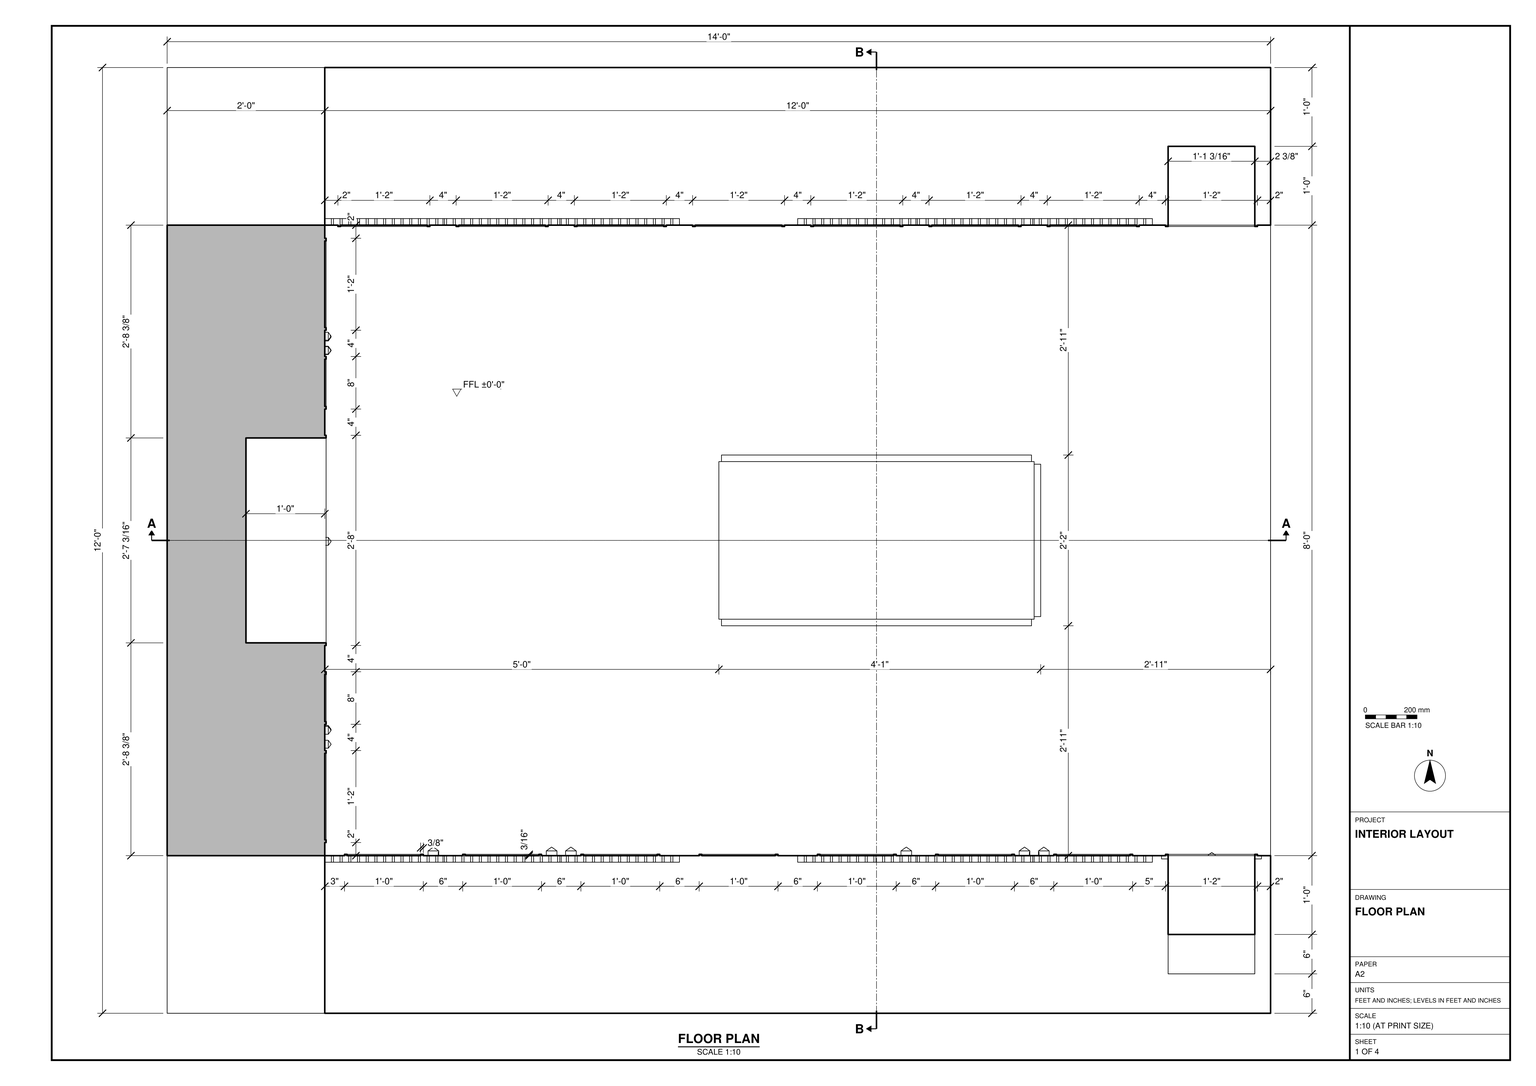
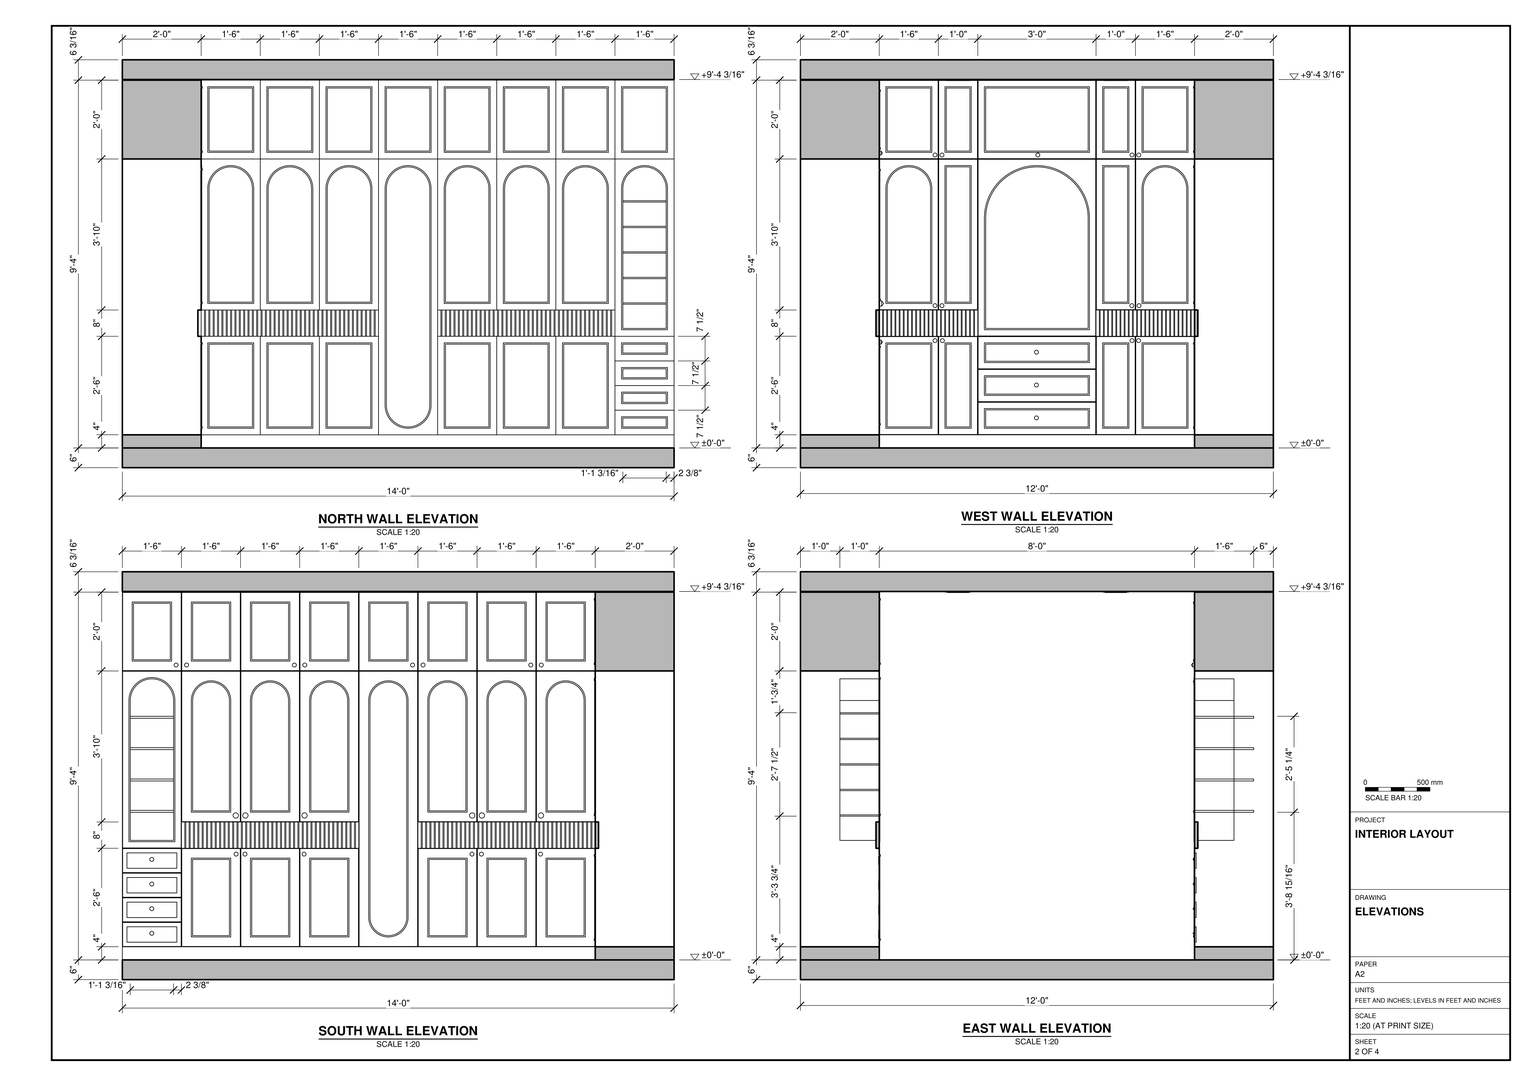
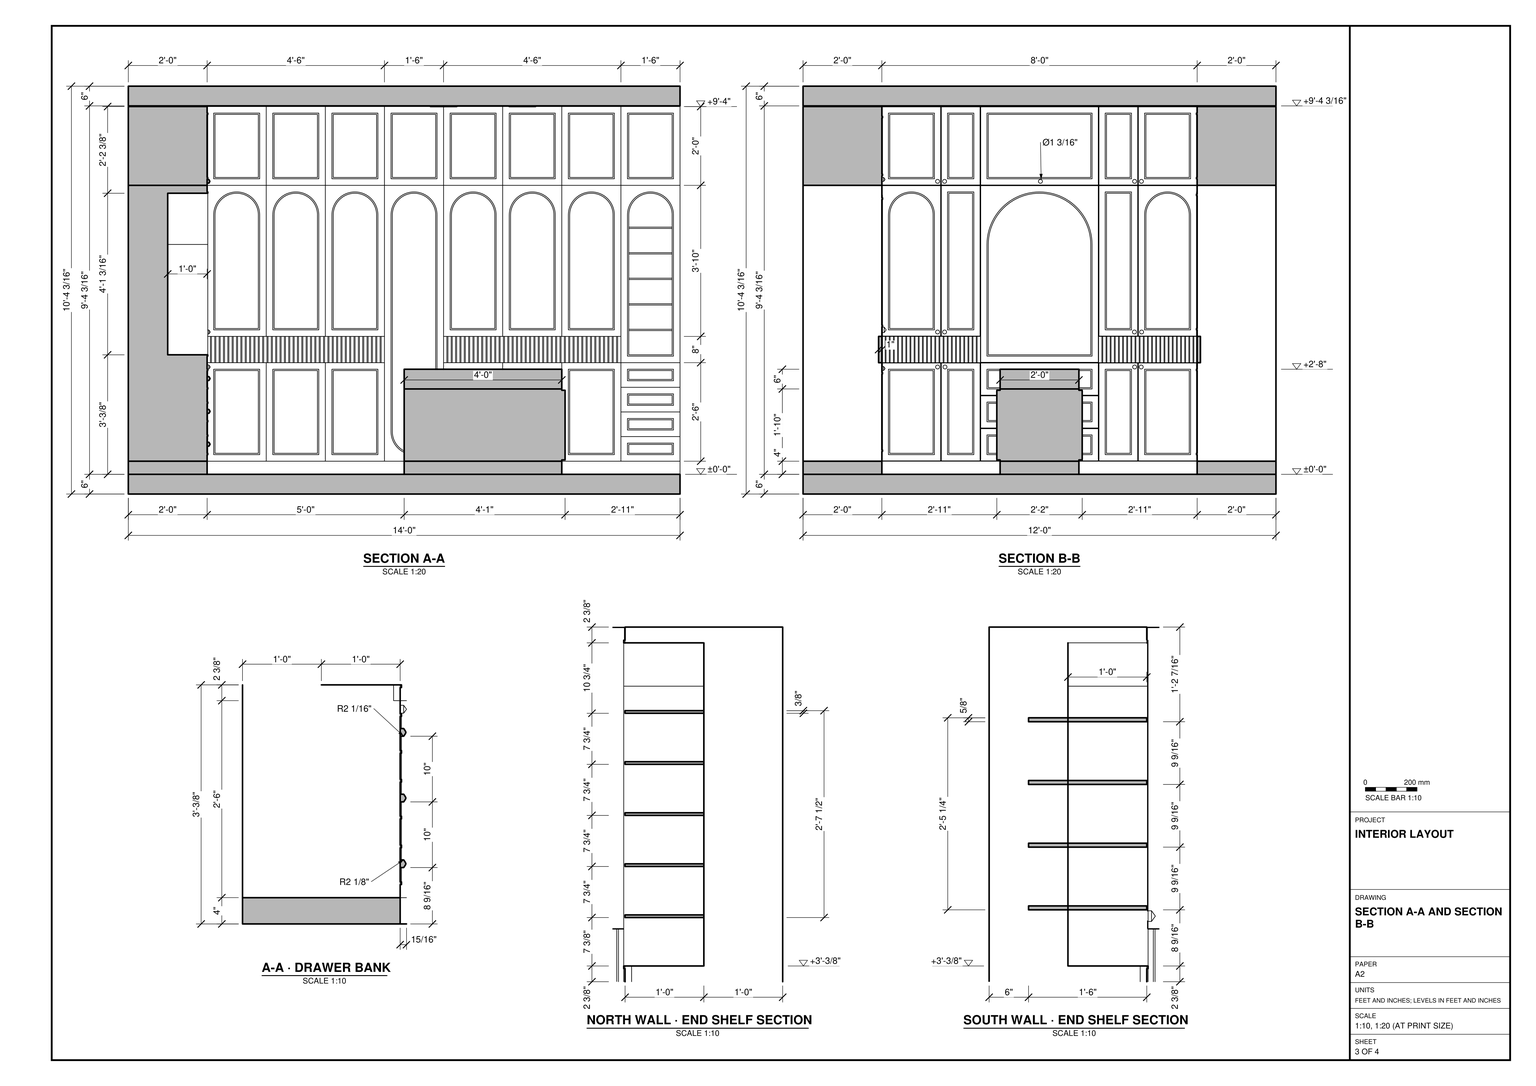
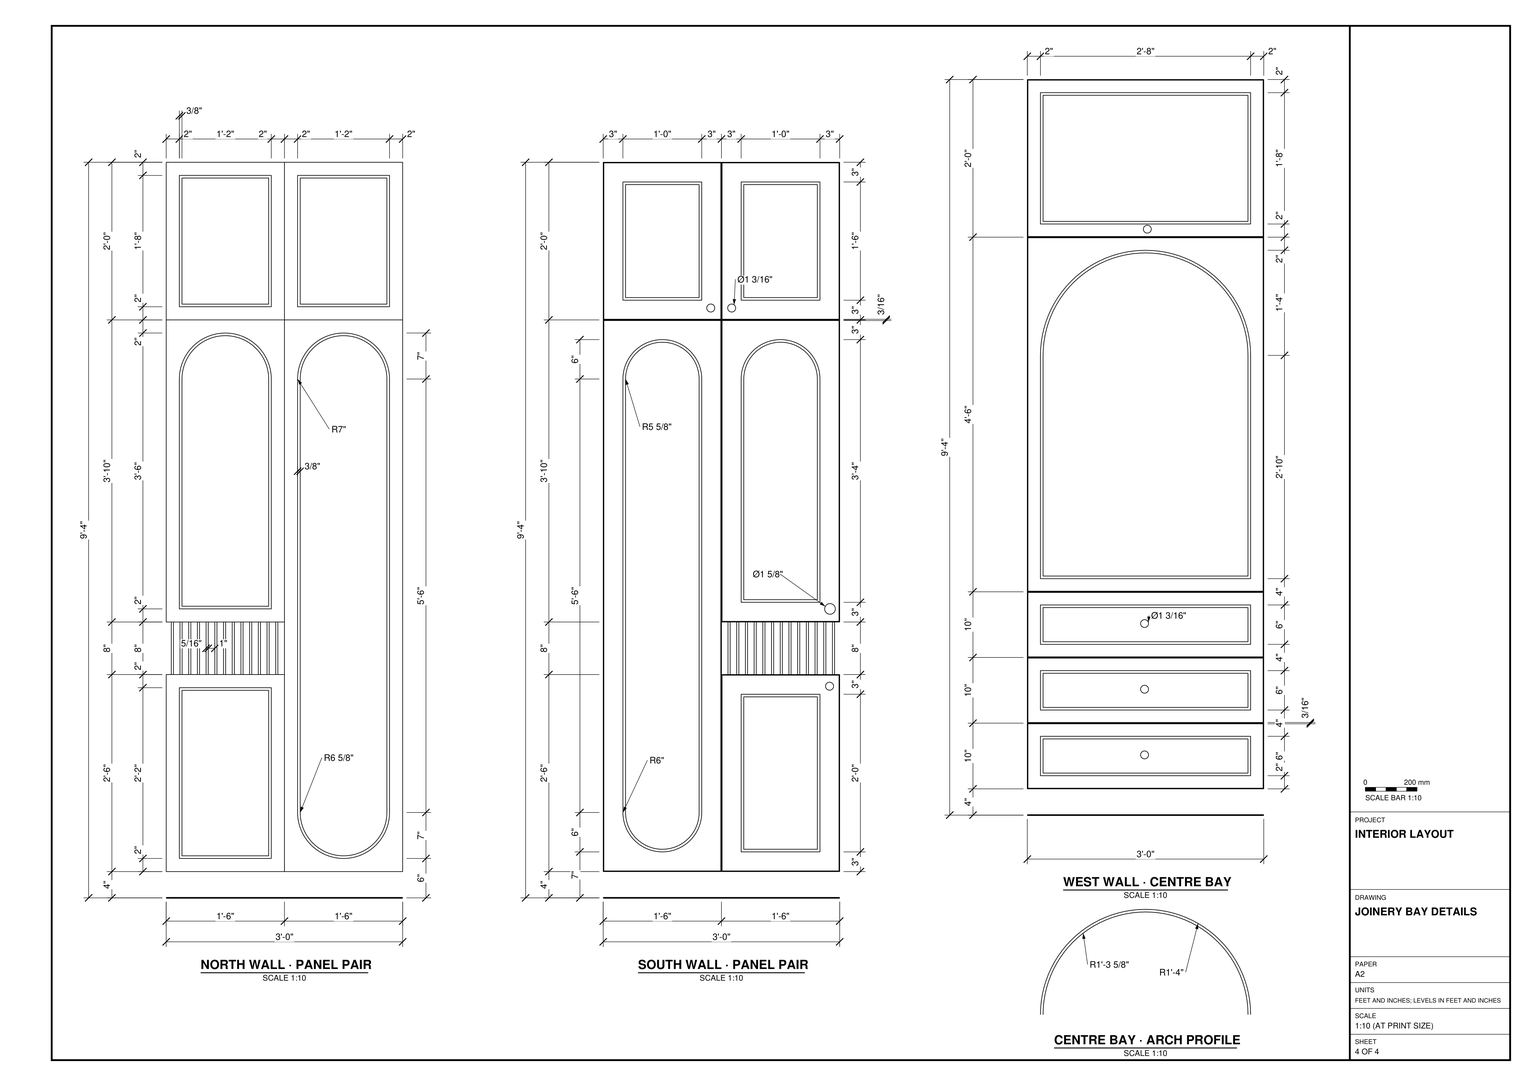
Build the dressing room in SketchUp from task_files/diagram_01.pdf. Work in feet and inches. The overall model is 14'-0" east to west, 12'-0" north to south and 10'-4 3/16" high. Use the single finished floor level of ±0'-0". Model the floor slab below that level and the ceiling slab above the cabinetry, following the thicknesses and edges in the sections.

Lay out the built-in storage along the north, south and west sides, leaving the east side clear between the ends of the long runs. On the north and south faces, align the upper cupboards, arched panels, ribbed bands and lower cupboards as shown in the elevations. Include the tall round-ended panel in each run and the shelved bay above a drawer stack at each east end. Follow the separate shelf sections rather than making the two end bays identical. On the west side, form the wider central arched recess over the drawer bank, with narrower cabinets to either side.

Model the freestanding island with its plinth, body and top. Use its overall footprint, rather than its plinth, to set the clearances shown in plan. Keep shell elements and individual furniture or joinery pieces in separate groups or components, and use components for repeated parts. Any decor or loose items shown may be suitable library components. Save one SketchUp model as output_files/walk_in_dressing_room_with_a_freestanding_island.skp.

# SketchUp Ruby script. Lengths in inches.
U = 1.inch
M = Sketchup.active_model
def pt(a) = Geom::Point3d.new(a.map { |v| v * U })
def face(e, loops, mat)
  f = e.add_face(loops[0].map { |a| pt(a) })
  loops[1..].each { |l| e.add_face(l.map { |a| pt(a) }).erase! }
  f.material = f.back_material = mat if mat
  f
end
# faces: each face lists its corners as indices into pts; further lists are holes
def faces(e, pts, list, mat = nil) = list.each { |f| face(e, (f[0].is_a?(Array) ? f : [f]).map { |l| l.map { |i| pts[i] } }, mat) }
# xy, xz, yz: faces in a plane at the given z, y or x. An outline is a flat list of corners, or four numbers for a rectangle; further outlines are holes
def ring(l) = l.size == 4 ? [[l[0], l[1]], [l[2], l[1]], [l[2], l[3]], [l[0], l[3]]] : l.each_slice(2).to_a
def flat(e, list, mat, &to3) = list.each { |f| face(e, (f[0].is_a?(Array) ? f : [f]).map { |l| ring(l).map { |u, v| to3.(u, v) } }, mat) }
def xy(e, z, list, mat = nil) = flat(e, list, mat) { |x, y| [x, y, z] }
def xz(e, y, list, mat = nil) = flat(e, list, mat) { |x, z| [x, y, z] }
def yz(e, x, list, mat = nil) = flat(e, list, mat) { |y, z| [x, y, z] }
def lines(e, pts, list) = list.each { |a, b| e.add_line(pt(pts[a]), pt(pts[b])) }
# prism: a flat outline (further loops are holes) pulled along v
def prism(e, loops, v, mat = nil)
  f = face(e, loops, mat); d = Geom::Vector3d.new(v.map { |x| x * U })
  f.pushpull(f.normal.samedirection?(d) ? d.length : -d.length)
end
def box(e, o, s, mat = nil) = prism(e, [[o, [o[0] + s[0], o[1], o[2]], [o[0] + s[0], o[1] + s[1], o[2]], [o[0], o[1] + s[1], o[2]]]], [0, 0, s[2]], mat)
def at(x, y, z, deg = 0) = Geom::Transformation.translation(pt([x, y, z])) * Geom::Transformation.rotation(ORIGIN, Z_AXIS, deg.degrees)
def axes(o, x, y, z) = Geom::Transformation.new([*x, 0, *y, 0, *z, 0, *pt(o).to_a, 1])
def part(name) = M.definitions.add(name)
# library, detail: a bought-in or finely detailed component or shape, given as its bounding box
def library(name, o, s) = part(name).tap { |d| box(d.entities, o, s) }
def detail(e, o, s) = box(e.add_group.entities, o, s)
def put(e, d, t, mat = nil) = e.add_instance(d, t).tap { |i| i.material = mat if mat }
def group(e, t, mat = nil) = e.add_group.tap { |g| g.transformation = t; g.material = mat if mat }.entities
root = M.entities
M.materials.add("[Translucent Glass Gray]1").color = [128, 128, 128]
M.materials.add("[Wood Veneer 01]").color = [104, 60, 32]
M.materials.add("download (3)").color = [228, 221, 207]
c1 = library("Group\#1",[0,0,0],[24.97,96,112])
c2 = part("Recessed ceiling light")
xy(c2.entities,0,[[4,0,2.96,0.14,2,0.54,1.17,1.17,0.54,2,0.14,2.96,0,4,0.14,5.04,0.54,6,1.17,6.83,2,7.46,2.96,7.86,4,8,5.04,7.86,6,7.46,6.83,6.83,7.46,6,7.86,5.04,8,4,7.86,2.96,7.46,2,6.83,1.17,6,0.54,5.04,0.14]])
xy(c2.entities,0.2,[[[4,0,5.04,0.14,6,0.54,6.83,1.17,7.46,2,7.86,2.96,8,4,7.86,5.04,7.46,6,6.83,6.83,6,7.46,5.04,7.86,4,8,2.96,7.86,2,7.46,1.17,6.83,0.54,6,0.14,5.04,0,4,0.14,2.96,0.54,2,1.17,1.17,2,0.54,2.96,0.14],[4,0.6,3.12,0.72,2.3,1.06,1.6,1.6,1.06,2.3,0.72,3.12,0.6,4,0.72,4.88,1.06,5.7,1.6,6.4,2.3,6.94,3.12,7.28,4,7.4,4.88,7.28,5.7,6.94,6.4,6.4,6.94,5.7,7.28,4.88,7.4,4,7.28,3.12,6.94,2.3,6.4,1.6,5.7,1.06,4.88,0.72]],[4,0.6,4.88,0.72,5.7,1.06,6.4,1.6,6.94,2.3,7.28,3.12,7.4,4,7.28,4.88,6.94,5.7,6.4,6.4,5.7,6.94,4.88,7.28,4,7.4,3.12,7.28,2.3,6.94,1.6,6.4,1.06,5.7,0.72,4.88,0.6,4,0.72,3.12,1.06,2.3,1.6,1.6,2.3,1.06,3.12,0.72]])
p = [[2.96,0.14,0],[4,0,0],[4,0,0.2],[2.96,0.14,0.2],[5.04,0.14,0],[5.04,0.14,0.2],
  [2,0.54,0],[2,0.54,0.2],[6,0.54,0],[6,0.54,0.2],[1.17,1.17,0],[1.17,1.17,0.2],
  [6.83,1.17,0],[6.83,1.17,0.2],[0.54,2,0],[0.54,2,0.2],[7.46,2,0],[7.46,2,0.2],
  [0.14,2.96,0],[0.14,2.96,0.2],[7.86,2.96,0],[7.86,2.96,0.2],[0,4,0],[0,4,0.2],
  [8,4,0],[8,4,0.2],[0.14,5.04,0],[0.14,5.04,0.2],[7.86,5.04,0],[7.86,5.04,0.2],
  [0.54,6,0],[0.54,6,0.2],[7.46,6,0],[7.46,6,0.2],[1.17,6.83,0],[1.17,6.83,0.2],
  [6.83,6.83,0],[6.83,6.83,0.2],[2,7.46,0],[2,7.46,0.2],[6,7.46,0],[6,7.46,0.2],
  [2.96,7.86,0],[2.96,7.86,0.2],[5.04,7.86,0],[5.04,7.86,0.2],[4,8,0],[4,8,0.2]]
faces(c2.entities,p,[[0,1,2,3],[1,4,5,2],[6,0,3,7],[4,8,9,5],[10,6,7,11],[8,12,13,9],[14,10,11,15],[12,16,17,13],
  [18,14,15,19],[16,20,21,17],[22,18,19,23],[20,24,25,21],[26,22,23,27],[24,28,29,25],[30,26,27,31],[28,32,33,29],
  [34,30,31,35],[32,36,37,33],[38,34,35,39],[36,40,41,37],[42,38,39,43],[40,44,45,41],[46,42,43,47],[44,46,47,45]])
c3 = part("Ceiling panel")
xy(c3.entities,0,[[0,0,0,144,168,144,168,120,24,120,24,24,168,24,168,0],[24,24,168,120]])
xy(c3.entities,6,[[0,0,168,144]])
xz(c3.entities,0,[[0,0,168,6]])
xz(c3.entities,144,[[0,0,168,6]])
yz(c3.entities,0,[[0,0,144,6]])
yz(c3.entities,168,[[0,0,144,6]])
c4 = library("Group\#18",[0,0,0],[144,24.2,112])
c5 = library("Group\#19",[0,0,0],[144,25.31,112])
put(root,c1,at(0,24,0))
g1 = group(root,at(84,60,0))
xy(g1,0,[[0,0,48,24]])
xy(g1,4,[[0,0,48,24]])
xy(g1,4.4,[[0.4,-1,47.6,0],[48,0.4,49,23.6],[0.4,24,47.6,25]],"[Wood Veneer 01]")
xy(g1,25.6,[[0.4,-1,47.6,0],[48,0.4,49,23.6],[0.4,24,47.6,25]],"[Wood Veneer 01]")
xy(g1,26,[[0,0,48,24]])
xy(g1,32,[[0,0,48,24]],"[Translucent Glass Gray]1")
xz(g1,-1,[[0.4,4.4,47.6,25.6]],"[Wood Veneer 01]")
xz(g1,0,[[0,26,48,32]],"[Translucent Glass Gray]1")
xz(g1,0,[[0,0,48,4],[[0,4,48,26],[0.4,4.4,47.6,25.6]]],"[Wood Veneer 01]")
xz(g1,0.4,[[48,4.4,49,25.6]],"[Wood Veneer 01]")
xz(g1,23.6,[[48,4.4,49,25.6]],"[Wood Veneer 01]")
xz(g1,24,[[0,26,48,32]],"[Translucent Glass Gray]1")
xz(g1,24,[[0,0,48,4],[[0,4,48,26],[0.4,4.4,47.6,25.6]]],"[Wood Veneer 01]")
xz(g1,25,[[0.4,4.4,47.6,25.6]],"[Wood Veneer 01]")
yz(g1,0,[[0,0,24,4],[0,4,24,26]])
yz(g1,0,[[0,26,24,32]],"[Translucent Glass Gray]1")
yz(g1,0.4,[[-1,4.4,0,25.6],[24,4.4,25,25.6]],"[Wood Veneer 01]")
yz(g1,47.6,[[-1,4.4,0,25.6],[24,4.4,25,25.6]],"[Wood Veneer 01]")
yz(g1,48,[[0,26,24,32]],"[Translucent Glass Gray]1")
yz(g1,48,[[0,0,24,4],[[0,4,24,26],[0.4,4.4,23.6,25.6]]],"[Wood Veneer 01]")
yz(g1,49,[[0.4,4.4,23.6,25.6]],"[Wood Veneer 01]")
g2 = group(root,at(24,0,-6))
box(g2,[-24,0,0],[168,144,6],"download (3)")
g3 = group(root,at(0,0,118.2))
put(g3,c2,axes([92,68,-6],[1,0,0],[0,1,0],[0,0,-1]))
put(g3,c2,axes([92,92,-6],[1,0,0],[0,1,0],[0,0,-1]))
put(g3,c2,axes([44,44,-6],[1,0,0],[0,1,0],[0,0,-1]))
put(g3,c2,axes([140,92,-6],[1,0,0],[0,1,0],[0,0,-1]))
put(g3,c2,axes([92,44,-6],[1,0,0],[0,1,0],[0,0,-1]))
put(g3,c2,axes([140,44,-6],[1,0,0],[0,1,0],[0,0,-1]))
put(g3,c3,axes([0,144,-6],[1,0,0],[0,-1,0],[0,0,1]))
put(g3,c2,axes([116,68,-6],[1,0,0],[0,1,0],[0,0,-1]))
put(g3,c2,axes([44,92,-6],[1,0,0],[0,1,0],[0,0,-1]))
put(root,c4,at(24,119.8,0))
put(root,c5,at(24,0,0))
